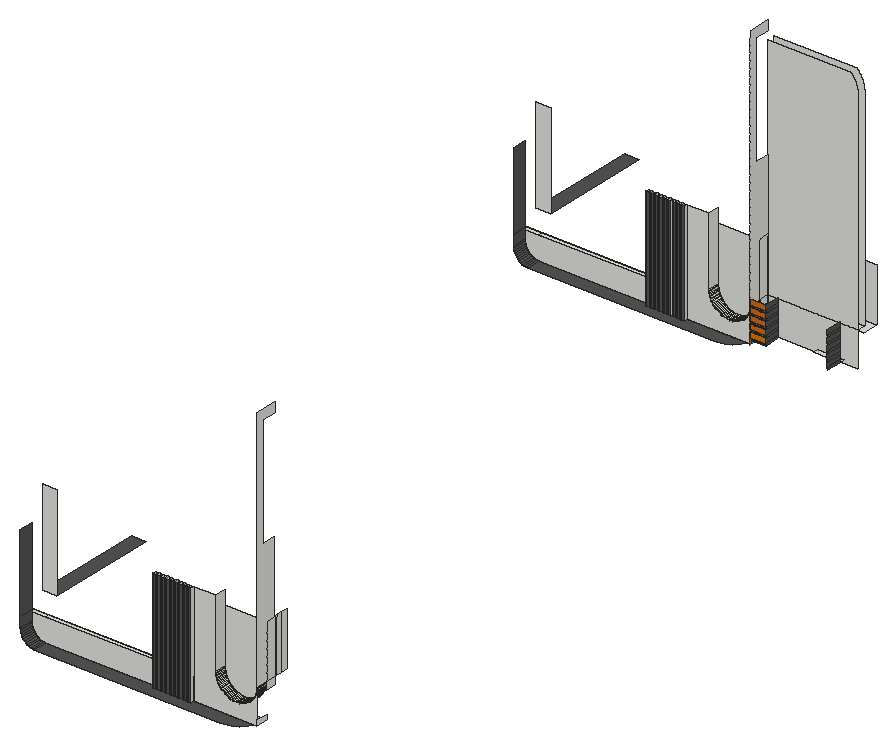
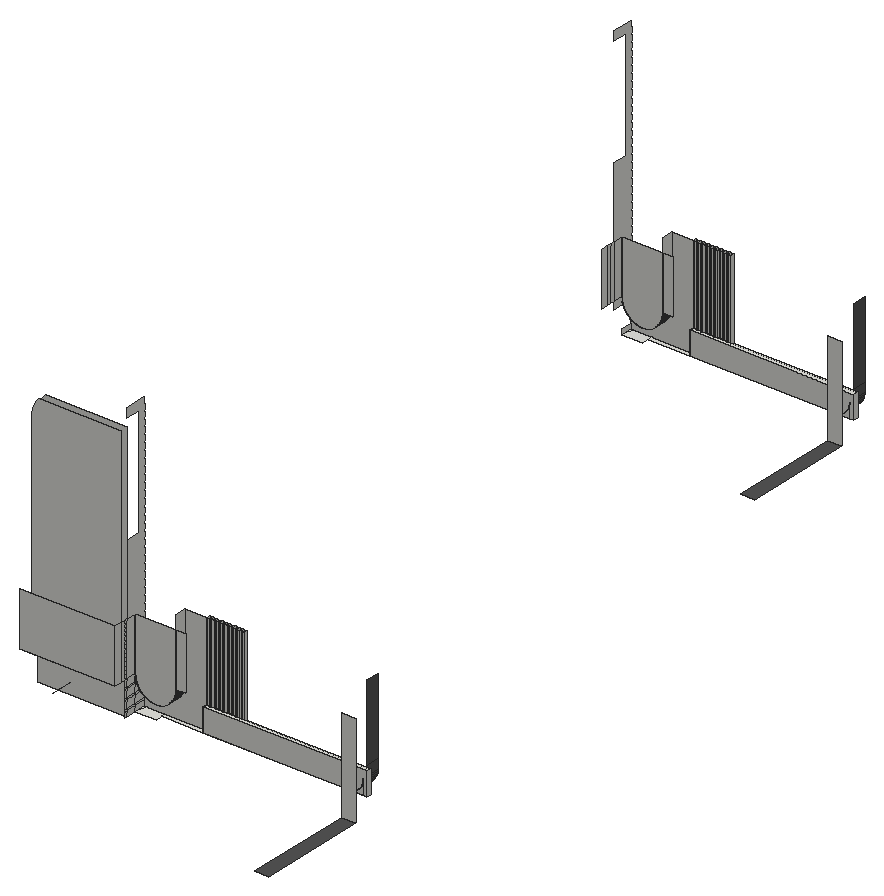
# SketchUp Ruby script. Lengths in inches.
U = 1.inch
M = Sketchup.active_model
def pt(a) = Geom::Point3d.new(a.map { |v| v * U })
def face(e, loops, mat)
  f = e.add_face(loops[0].map { |a| pt(a) })
  loops[1..].each { |l| e.add_face(l.map { |a| pt(a) }).erase! }
  f.material = f.back_material = mat if mat
  f
end
# faces: each face lists its corners as indices into pts; further lists are holes
def faces(e, pts, list, mat = nil) = list.each { |f| face(e, (f[0].is_a?(Array) ? f : [f]).map { |l| l.map { |i| pts[i] } }, mat) }
# xy, xz, yz: faces in a plane at the given z, y or x. An outline is a flat list of corners, or four numbers for a rectangle; further outlines are holes
def ring(l) = l.size == 4 ? [[l[0], l[1]], [l[2], l[1]], [l[2], l[3]], [l[0], l[3]]] : l.each_slice(2).to_a
def flat(e, list, mat, &to3) = list.each { |f| face(e, (f[0].is_a?(Array) ? f : [f]).map { |l| ring(l).map { |u, v| to3.(u, v) } }, mat) }
def xy(e, z, list, mat = nil) = flat(e, list, mat) { |x, y| [x, y, z] }
def xz(e, y, list, mat = nil) = flat(e, list, mat) { |x, z| [x, y, z] }
def yz(e, x, list, mat = nil) = flat(e, list, mat) { |y, z| [x, y, z] }
def lines(e, pts, list) = list.each { |a, b| e.add_line(pt(pts[a]), pt(pts[b])) }
# prism: a flat outline (further loops are holes) pulled along v
def prism(e, loops, v, mat = nil)
  f = face(e, loops, mat); d = Geom::Vector3d.new(v.map { |x| x * U })
  f.pushpull(f.normal.samedirection?(d) ? d.length : -d.length)
end
def box(e, o, s, mat = nil) = prism(e, [[o, [o[0] + s[0], o[1], o[2]], [o[0] + s[0], o[1] + s[1], o[2]], [o[0], o[1] + s[1], o[2]]]], [0, 0, s[2]], mat)
def at(x, y, z, deg = 0) = Geom::Transformation.translation(pt([x, y, z])) * Geom::Transformation.rotation(ORIGIN, Z_AXIS, deg.degrees)
def axes(o, x, y, z) = Geom::Transformation.new([*x, 0, *y, 0, *z, 0, *pt(o).to_a, 1])
def part(name) = M.definitions.add(name)
# library, detail: a bought-in or finely detailed component or shape, given as its bounding box
def library(name, o, s) = part(name).tap { |d| box(d.entities, o, s) }
def detail(e, o, s) = box(e.add_group.entities, o, s)
def put(e, d, t, mat = nil) = e.add_instance(d, t).tap { |i| i.material = mat if mat }
def group(e, t, mat = nil) = e.add_group.tap { |g| g.transformation = t; g.material = mat if mat }.entities
root = M.entities
M.materials.add("[0039_DarkOrange]").color = [219, 120, 0]
M.materials.add("[0041_Chocolate]").color = [210, 105, 30]
M.materials.add("[Color M06]").color = [84, 84, 84]
xy(root,141.26,[[675.54,281.47,692.98,285.84],[692.98,281.47,836,285.84],[836,281.47,876.59,285.84],[876.59,281.47,894.57,281.47,895.33,283,896.37,286.06,897,289.23,897.21,292.45,876.59,292.45],[894.57,281.47,895.33,283,896.37,286.06,897,289.23,897.21,292.45,897.21,281.47],
  [598.85,972.36,616.29,976.74],[616.29,972.36,759.32,976.74],[759.32,972.36,799.9,976.74],[799.9,972.36,817.89,972.36,818.64,973.89,819.68,976.95,820.3125,980.12,820.52,983.34,799.9,983.34],[817.89,972.36,818.64,973.89,819.68,976.95,820.3125,980.12,820.52,983.34,820.52,972.36]])
xy(root,141.26,[[692.98,267.75,872.51,267.75,875.73,267.96,878.9,268.59,881.96,269.63,884.86,271.06,887.55,272.85,889.98,274.98,892.11,277.41,893.9,280.1,894.57,281.47,836,281.47,836,278.34,832.88,278.34,832.88,281.47,831.63,281.47,831.63,278.34,828.5,278.34,828.5,281.47,827.44,281.47,827.44,278.34,824.32,278.34,824.32,281.47,823.25,281.47,823.25,278.34,820.13,278.34,820.13,281.47,819.07,281.47,819.07,278.34,815.94,278.34,815.94,281.47,814.88,281.47,814.88,278.34,811.75,278.34,811.75,281.47,810.63,281.47,810.63,278.34,807.5,278.34,807.5,281.47,806.38,281.47,806.38,278.34,803.25,278.34,803.25,281.47,802.13,281.47,802.13,278.34,799,278.34,799,281.47,692.98,281.47],[616.29,958.64,795.82,958.64,799.05,958.86,802.22,959.49,805.28,960.52,808.17,961.95,810.86,963.75,813.29,965.88,815.42,968.31,817.21,970.99,817.89,972.36,759.32,972.36,759.32,969.24,756.19,969.24,756.19,972.36,754.94,972.36,754.94,969.24,751.82,969.24,751.82,972.36,750.75,972.36,750.75,969.24,747.63,969.24,747.63,972.36,746.57,972.36,746.57,969.24,743.44,969.24,743.44,972.36,742.38,972.36,742.38,969.24,739.25,969.24,739.25,972.36,738.19,972.36,738.19,969.24,735.07,969.24,735.07,972.36,733.94,972.36,733.94,969.24,730.82,969.24,730.82,972.36,729.69,972.36,729.69,969.24,726.57,969.24,726.57,972.36,725.44,972.36,725.44,969.24,722.32,969.24,722.32,972.36,616.29,972.36]],"[Color M06]")
xy(root,145.27,[[870.3,986.55,895.48,991.24]])
xy(root,145.27,[[820.52,971.36,835.91,972.36]],"[0039_DarkOrange]")
xy(root,147.375,[[820.52,971.36,835.91,972.36]],"[0039_DarkOrange]")
xy(root,148.66,[[648.9,333.33,662.61,439.98],[572.21,1024.22,585.93,1130.875]],"[Color M06]")
xy(root,152.33,[[820.52,971.36,835.91,972.36]],"[0039_DarkOrange]")
xy(root,154.4375,[[820.52,971.36,835.91,972.36]],"[0041_Chocolate]")
xy(root,159.39,[[820.52,971.36,835.91,972.36]],"[0041_Chocolate]")
xy(root,161.5,[[820.52,971.36,835.91,972.36]],"[0041_Chocolate]")
xy(root,163.7,[[675.54,281.47,692.98,285.84],[692.98,281.47,836,285.84],[598.85,972.36,616.29,976.74],[616.29,972.36,759.32,976.74]])
xy(root,166.45,[[820.52,971.36,835.91,972.36]],"[0041_Chocolate]")
xy(root,168.5625,[[820.52,971.36,835.91,972.36]],"[0041_Chocolate]")
xy(root,173.52,[[820.52,971.36,835.91,972.36]],"[0041_Chocolate]")
xy(root,174.51,[[820.52,993.35,907.49,1001.16],[907.49,993.35,907.49,1001.16,820.52,1001.16,820.52,1008.21,913.34,1008.21,913.34,993.35]])
xy(root,175.625,[[820.52,971.36,835.91,972.36]],"[0041_Chocolate]")
xz(root,278.34,[[799,141.26,802.13,240.16],[803.25,141.26,806.38,240.16],[807.5,141.26,810.63,240.16],[811.75,141.26,814.88,240.16],[815.94,141.26,819.07,240.16],
  [820.13,141.26,823.25,240.16],[824.32,141.26,827.44,240.16],[828.5,141.26,831.63,240.16],[832.88,141.26,836,240.16]],"[Color M06]")
xz(root,281.47,[[675.54,141.26,679.54,163.7],[679.54,141.26,692.98,141.26,691.2,141.46,689.46,141.89,687.79,142.53,686.21,143.38,684.75,144.42,683.43,145.64,682.28,147.01,681.32,148.52,680.55,150.14,679.99,151.84,679.65,153.6,679.54,155.39],[692.98,141.26,799,141.26,799,163.7,679.54,163.7,679.54,155.39,679.65,153.6,679.99,151.84,680.55,150.14,681.32,148.52,682.28,147.01,683.43,145.64,684.75,144.42,686.21,143.38,687.79,142.53,689.46,141.89,691.2,141.46],[799,141.26,802.13,163.7],[802.13,141.26,803.25,163.7],
  [803.25,141.26,806.38,163.7],[806.38,141.26,807.5,163.7],[807.5,141.26,810.63,163.7],[810.63,141.26,811.75,163.7],[811.75,141.26,814.88,163.7],
  [814.88,141.26,815.94,163.7],[815.94,141.26,819.07,163.7],[819.07,141.26,820.13,163.7],[820.13,141.26,823.25,163.7],[823.25,141.26,824.32,163.7],
  [824.32,141.26,827.44,163.7],[827.44,141.26,828.5,163.7],[828.5,141.26,831.63,163.7],[831.63,141.26,832.88,163.7],[832.88,141.26,836,163.7],
  [836,141.26,897.21,141.26,897.21,174.51,897.18,173.46,897.1,172.42,896.96,171.38,896.77,170.36,896.53,169.34,896.23,168.33,895.88,167.35,895.48,166.38,895.03,165.4375,894.53,164.52,893.99,163.625,893.39,162.76,892.76,161.93,892.08,161.14,891.36,160.38,890.6,159.66,889.8,158.98,888.97,158.34,888.11,157.75,887.22,157.2,886.3,156.7,885.36,156.25,884.39,155.85,883.4,155.5,882.4,155.21,881.38,154.96,880.35,154.77,879.32,154.64,878.27,154.55,877.23,154.53,876.18,154.55,875.14,154.64,874.1,154.77,873.07,154.96,872.05,155.21,871.05,155.5,870.07,155.85,869.1,156.25,868.15,156.7,867.23,157.2,866.34,157.75,865.48,158.34,864.65,158.98,863.85,159.66,863.1,160.38,862.375,161.14,861.7,161.93,861.06,162.76,860.47,163.625,859.92,164.52,859.42,165.4375,858.97,166.38,858.57,167.35,858.22,168.33,857.92,169.34,857.68,170.36,857.49,171.38,857.35,172.42,857.27,173.46,857.24,174.51,857.24,240.16,836,240.16],[799,163.7,802.13,240.16],[803.25,163.7,806.38,240.16],[807.5,163.7,810.63,240.16],[811.75,163.7,814.88,240.16],
  [815.94,163.7,819.07,240.16],[820.13,163.7,823.25,240.16],[824.32,163.7,827.44,240.16],[828.5,163.7,831.63,240.16],[832.88,163.7,836,240.16]])
xz(root,285.84,[[675.54,141.26,675.54,163.7,692.98,163.7,692.98,141.26,691.2,141.46,689.46,141.89,687.79,142.53,686.21,143.38,684.75,144.42,683.43,145.64,682.28,147.01,681.32,148.52,680.55,150.14,679.99,151.84,679.65,153.6,679.54,155.39,679.54,141.26],[679.54,141.26,679.54,155.39,679.65,153.6,679.99,151.84,680.55,150.14,681.32,148.52,682.28,147.01,683.43,145.64,684.75,144.42,686.21,143.38,687.79,142.53,689.46,141.89,691.2,141.46,692.98,141.26],[692.98,141.26,836,163.7]])
xz(root,292.45,[[877.23,154.53,878.27,154.55,879.32,154.64,880.35,154.77,881.38,154.96,882.4,155.21,883.4,155.5,884.39,155.85,885.36,156.25,886.3,156.7,887.22,157.2,888.11,157.75,888.97,158.34,889.8,158.98,890.6,159.66,891.36,160.38,892.08,161.14,892.76,161.93,893.39,162.76,893.99,163.625,894.53,164.52,895.03,165.4375,895.48,166.38,895.88,167.35,896.23,168.33,896.53,169.34,896.77,170.36,896.96,171.38,897.1,172.42,897.18,173.46,897.21,174.51,897.21,226.8,857.24,226.8,857.24,174.51,857.27,173.46,857.35,172.42,857.49,171.38,857.68,170.36,857.92,169.34,858.22,168.33,858.57,167.35,858.97,166.38,859.42,165.4375,859.92,164.52,860.47,163.625,861.06,162.76,861.7,161.93,862.375,161.14,863.1,160.38,863.85,159.66,864.65,158.98,865.48,158.34,866.34,157.75,867.23,157.2,868.15,156.7,869.1,156.25,870.07,155.85,871.05,155.5,872.05,155.21,873.07,154.96,874.1,154.77,875.14,154.64,876.18,154.55],[847.59,174.51,857.24,226.8]])
xz(root,333.33,[[648.9,148.66,662.61,240.16]])
xz(root,969.24,[[722.32,141.26,725.44,240.16],[726.57,141.26,729.69,240.16],[730.82,141.26,733.94,240.16],[735.07,141.26,738.19,240.16],[739.25,141.26,742.38,240.16],
  [743.44,141.26,746.57,240.16],[747.63,141.26,750.75,240.16],[751.82,141.26,754.94,240.16],[756.19,141.26,759.32,240.16]],"[Color M06]")
xz(root,971.36,[[820.52,147.375,835.91,152.33]],"[0039_DarkOrange]")
xz(root,971.36,[[820.52,154.4375,835.91,159.39],[820.52,161.5,835.91,166.45],[820.52,168.5625,835.91,173.52],[820.52,175.625,835.91,180.58]],"[0041_Chocolate]")
xz(root,972.36,[[598.85,141.26,602.85,163.7],[602.85,141.26,616.29,141.26,614.51,141.46,612.77,141.89,611.1,142.53,609.52,143.38,608.0625,144.42,606.75,145.64,605.6,147.01,604.63,148.52,603.86,150.14,603.3,151.84,602.96,153.6,602.85,155.39],[616.29,141.26,722.32,141.26,722.32,163.7,602.85,163.7,602.85,155.39,602.96,153.6,603.3,151.84,603.86,150.14,604.63,148.52,605.6,147.01,606.75,145.64,608.0625,144.42,609.52,143.38,611.1,142.53,612.77,141.89,614.51,141.46],[722.32,141.26,725.44,163.7],[725.44,141.26,726.57,163.7],
  [726.57,141.26,729.69,163.7],[729.69,141.26,730.82,163.7],[730.82,141.26,733.94,163.7],[733.94,141.26,735.07,163.7],[735.07,141.26,738.19,163.7],
  [738.19,141.26,739.25,163.7],[739.25,141.26,742.38,163.7],[742.38,141.26,743.44,163.7],[743.44,141.26,746.57,163.7],[746.57,141.26,747.63,163.7],
  [747.63,141.26,750.75,163.7],[750.75,141.26,751.82,163.7],[751.82,141.26,754.94,163.7],[754.94,141.26,756.19,163.7],[756.19,141.26,759.32,163.7],
  [759.32,141.26,820.52,141.26,820.52,174.51,820.5,173.46,820.41,172.42,820.28,171.38,820.09,170.36,819.84,169.34,819.55,168.33,819.2,167.35,818.8,166.38,818.35,165.4375,817.85,164.52,817.3,163.625,816.71,162.76,816.07,161.93,815.39,161.14,814.67,160.38,813.91,159.66,813.12,158.98,812.29,158.34,811.42,157.75,810.53,157.2,809.61,156.7,808.67,156.25,807.7,155.85,806.71,155.5,805.71,155.21,804.69,154.96,803.67,154.77,802.63,154.64,801.59,154.55,800.54,154.53,799.49,154.55,798.45,154.64,797.41,154.77,796.38,154.96,795.37,155.21,794.36,155.5,793.38,155.85,792.41,156.25,791.47,156.7,790.55,157.2,789.66,157.75,788.79,158.34,787.96,158.98,787.17,159.66,786.41,160.38,785.6875,161.14,785.01,161.93,784.37,162.76,783.78,163.625,783.23,164.52,782.73,165.4375,782.28,166.38,781.88,167.35,781.53,168.33,781.24,169.34,780.99,170.36,780.8,171.38,780.66,172.42,780.58,173.46,780.56,174.51,780.56,240.16,759.32,240.16],[722.32,163.7,725.44,240.16],[726.57,163.7,729.69,240.16],[730.82,163.7,733.94,240.16],[735.07,163.7,738.19,240.16],
  [739.25,163.7,742.38,240.16],[743.44,163.7,746.57,240.16],[747.63,163.7,750.75,240.16],[751.82,163.7,754.94,240.16],[756.19,163.7,759.32,240.16]])
xz(root,972.36,[[820.52,145.27,835.91,147.375]],"[0039_DarkOrange]")
xz(root,972.36,[[820.52,152.33,835.91,154.4375],[820.52,159.39,835.91,161.5],[820.52,166.45,835.91,168.5625],[820.52,173.52,835.91,175.625]],"[0041_Chocolate]")
xz(root,976.74,[[598.85,141.26,598.85,163.7,616.29,163.7,616.29,141.26,614.51,141.46,612.77,141.89,611.1,142.53,609.52,143.38,608.0625,144.42,606.75,145.64,605.6,147.01,604.63,148.52,603.86,150.14,603.3,151.84,602.96,153.6,602.85,155.39,602.85,141.26],[602.85,141.26,602.85,155.39,602.96,153.6,603.3,151.84,603.86,150.14,604.63,148.52,605.6,147.01,606.75,145.64,608.0625,144.42,609.52,143.38,611.1,142.53,612.77,141.89,614.51,141.46,616.29,141.26],[616.29,141.26,759.32,163.7]])
xz(root,983.34,[[800.54,154.53,801.59,154.55,802.63,154.64,803.67,154.77,804.69,154.96,805.71,155.21,806.71,155.5,807.7,155.85,808.67,156.25,809.61,156.7,810.53,157.2,811.42,157.75,812.29,158.34,813.12,158.98,813.91,159.66,814.67,160.38,815.39,161.14,816.07,161.93,816.71,162.76,817.3,163.625,817.85,164.52,818.35,165.4375,818.8,166.38,819.2,167.35,819.55,168.33,819.84,169.34,820.09,170.36,820.28,171.38,820.41,172.42,820.5,173.46,820.52,174.51,820.52,226.8,780.56,226.8,780.56,174.51,780.58,173.46,780.66,172.42,780.8,171.38,780.99,170.36,781.24,169.34,781.53,168.33,781.88,167.35,782.28,166.38,782.73,165.4375,783.23,164.52,783.78,163.625,784.37,162.76,785.01,161.93,785.6875,161.14,786.41,160.38,787.17,159.66,787.96,158.98,788.79,158.34,789.66,157.75,790.55,157.2,791.47,156.7,792.41,156.25,793.38,155.85,794.36,155.5,795.37,155.21,796.38,154.96,797.41,154.77,798.45,154.64,799.49,154.55],[770.9,174.51,780.56,226.8]])
xz(root,993.35,[[820.52,141.26,907.49,174.51],[820.52,174.51,907.49,174.51,907.49,376.875,907.48,377.55,907.46,378.22,907.41,378.9,907.35,379.57,907.27,380.24,907.17,380.9,907.06,381.57,906.93,382.23,906.78,382.89,906.61,383.54,906.59,383.64,906.43,384.19,906.23,384.84,906.01,385.47,905.91,385.76,905.78,386.11,905.53,386.73,905.26,387.35,904.98,387.96,904.68,388.57,904.37,389.17,904.04,389.76,903.7,390.33,903.34,390.9,902.96,391.47,902.57,392.02,902.17,392.56,901.75,393.09,901.71,393.14,901.32,393.6,900.875,394.11,900.42,394.61,899.95,395.09,899.77,395.26,820.52,395.26]])
xz(root,1001.16,[[820.52,174.51,820.52,395.26,899.77,395.26,899.95,395.09,900.42,394.61,900.875,394.11,901.32,393.6,901.71,393.14,901.75,393.09,902.17,392.56,902.57,392.02,902.96,391.47,903.34,390.9,903.7,390.33,904.04,389.76,904.37,389.17,904.68,388.57,904.98,387.96,905.26,387.35,905.53,386.73,905.78,386.11,905.91,385.76,906.01,385.47,906.23,384.84,906.43,384.19,906.59,383.64,906.61,383.54,906.78,382.89,906.93,382.23,907.06,381.57,907.17,380.9,907.27,380.24,907.35,379.57,907.41,378.9,907.46,378.22,907.48,377.55,907.49,376.875,907.49,174.51]])
xz(root,1008.21,[[820.52,174.51,913.34,226.8]])
xz(root,1024.22,[[572.21,148.66,585.93,240.16]])
yz(root,598.85,[[972.36,141.26,976.74,163.7]])
yz(root,602.85,[[958.64,155.39,972.36,164.97],[958.64,164.97,972.36,240.16]],"[Color M06]")
yz(root,675.54,[[281.47,141.26,285.84,163.7]])
yz(root,679.54,[[267.75,155.39,281.47,164.97],[267.75,164.97,281.47,240.16]],"[Color M06]")
yz(root,722.32,[[969.24,141.26,972.36,240.16]])
yz(root,725.44,[[969.24,141.26,972.36,240.16]])
yz(root,726.57,[[969.24,141.26,972.36,240.16]])
yz(root,729.69,[[969.24,141.26,972.36,240.16]])
yz(root,730.82,[[969.24,141.26,972.36,240.16]])
yz(root,733.94,[[969.24,141.26,972.36,240.16]])
yz(root,735.07,[[969.24,141.26,972.36,240.16]])
yz(root,738.19,[[969.24,141.26,972.36,240.16]])
yz(root,739.25,[[969.24,141.26,972.36,240.16]])
yz(root,742.38,[[969.24,141.26,972.36,240.16]])
yz(root,743.44,[[969.24,141.26,972.36,240.16]])
yz(root,746.57,[[969.24,141.26,972.36,240.16]])
yz(root,747.63,[[969.24,141.26,972.36,240.16]])
yz(root,750.75,[[969.24,141.26,972.36,240.16]])
yz(root,751.82,[[969.24,141.26,972.36,240.16]])
yz(root,754.94,[[969.24,141.26,972.36,240.16]])
yz(root,756.19,[[969.24,141.26,972.36,240.16]])
yz(root,759.32,[[969.24,141.26,972.36,240.16],[972.36,141.26,976.74,163.7]])
yz(root,780.56,[[972.36,174.51,983.34,240.16]])
yz(root,799,[[278.34,141.26,281.47,240.16]])
yz(root,802.13,[[278.34,141.26,281.47,240.16]])
yz(root,803.25,[[278.34,141.26,281.47,240.16]])
yz(root,806.38,[[278.34,141.26,281.47,240.16]])
yz(root,807.5,[[278.34,141.26,281.47,240.16]])
yz(root,810.63,[[278.34,141.26,281.47,240.16]])
yz(root,811.75,[[278.34,141.26,281.47,240.16]])
yz(root,814.88,[[278.34,141.26,281.47,240.16]])
yz(root,815.94,[[278.34,141.26,281.47,240.16]])
yz(root,819.07,[[278.34,141.26,281.47,240.16]])
yz(root,820.13,[[278.34,141.26,281.47,240.16]])
yz(root,820.52,[[972.36,141.26,983.34,146.14],[983.34,141.26,993.35,146.14],[993.35,141.26,996.48,146.14],[972.36,146.14,983.34,148.26],[983.34,146.14,993.35,148.26],
  [993.35,146.14,996.48,148.26],[972.36,148.26,983.34,155.64],[983.34,148.26,993.35,155.64],[993.35,148.26,996.48,155.64],[972.36,155.64,983.34,157.76],
  [983.34,155.64,993.35,157.76],[993.35,155.64,996.48,157.76],[972.36,157.76,983.34,165.14],[983.34,157.76,993.35,165.14],[993.35,157.76,996.48,165.14],
  [972.36,165.14,983.34,167.26],[983.34,165.14,993.35,167.26],[993.35,165.14,996.48,167.26],[972.36,167.26,983.34,174.51],[983.34,167.26,993.35,174.51],
  [993.35,167.26,996.48,174.51],[972.36,174.51,972.36,175.625,971.36,175.625,971.36,180.58,972.36,180.58,972.36,182.6875,971.36,182.6875,971.36,187.64,972.36,187.64,972.36,189.75,971.36,189.75,971.36,194.7,972.36,194.7,972.36,196.8125,971.36,196.8125,971.36,201.77,972.36,201.77,972.36,203.875,971.36,203.875,971.36,208.83,972.36,208.83,972.36,210.9375,971.36,210.9375,971.36,215.89,972.36,215.89,972.36,218,971.36,218,971.36,222.95,972.36,222.95,972.36,225.0625,971.36,225.0625,971.36,230.02,972.36,230.02,972.36,232.125,971.36,232.125,971.36,237.08,972.36,237.08,972.36,239.1875,971.36,239.1875,971.36,244.14,972.36,244.14,972.36,246.25,971.36,246.25,971.36,251.2,972.36,251.2,972.36,253.3125,971.36,253.3125,971.36,258.27,972.36,258.27,972.36,260.375,971.36,260.375,971.36,265.33,972.36,265.33,972.36,267.4375,971.36,267.4375,971.36,272.39,972.36,272.39,972.36,274.5,971.36,274.5,971.36,279.45,972.36,279.45,972.36,281.5625,971.36,281.5625,971.36,286.52,972.36,286.52,972.36,288.625,971.36,288.625,971.36,293.58,972.36,293.58,972.36,295.6875,971.36,295.6875,971.36,300.64,972.36,300.64,972.36,302.75,971.36,302.75,971.36,307.7,972.36,307.7,972.36,309.8125,971.36,309.8125,971.36,314.77,972.36,314.77,972.36,316.875,971.36,316.875,971.36,321.83,972.36,321.83,972.36,323.9375,971.36,323.9375,971.36,328.89,972.36,328.89,972.36,331,971.36,331,971.36,335.95,972.36,335.95,972.36,338.0625,971.36,338.0625,971.36,343.02,972.36,343.02,972.36,345.125,971.36,345.125,971.36,350.08,972.36,350.08,972.36,352.1875,971.36,352.1875,971.36,357.14,972.36,357.14,972.36,359.25,971.36,359.25,971.36,364.2,972.36,364.2,972.36,366.3125,971.36,366.3125,971.36,371.27,972.36,371.27,972.36,373.1875,971.36,373.1875,971.36,378.14,972.36,378.14,972.36,380.0625,971.36,380.0625,971.36,385.02,972.36,385.02,972.36,386.9375,971.36,386.9375,971.36,391.89,972.36,391.89,972.36,393.8125,971.36,393.8125,971.36,398.77,972.36,398.77,972.36,400.6875,971.36,400.6875,971.36,405.64,972.36,405.64,972.36,411.82,993.35,411.82,993.35,402.64,978.84,402.64,978.84,295.72,992.96,295.72,992.96,226.8,983.34,226.8,983.34,174.51],[983.34,174.51,993.35,226.8],[993.35,174.51,996.48,226.8],[996.48,174.51,1001.16,226.8],
  [1001.16,174.51,1008.21,226.8]])
yz(root,820.52,[[971.36,141.26,972.36,145.27],[971.36,147.375,972.36,148.26],[971.36,148.26,972.36,152.33]],"[0039_DarkOrange]")
yz(root,820.52,[[971.36,154.4375,972.36,155.64],[971.36,155.64,972.36,157.76],[971.36,157.76,972.36,159.39],[971.36,161.5,972.36,165.14],[971.36,165.14,972.36,166.45],
  [971.36,168.5625,972.36,173.52]],"[0041_Chocolate]")
yz(root,823.25,[[278.34,141.26,281.47,240.16]])
yz(root,824.32,[[278.34,141.26,281.47,240.16]])
yz(root,827.44,[[278.34,141.26,281.47,240.16]])
yz(root,828.5,[[278.34,141.26,281.47,240.16]])
yz(root,831.63,[[278.34,141.26,281.47,240.16]])
yz(root,832.88,[[278.34,141.26,281.47,240.16]])
yz(root,835.91,[[972.36,145.27,986.55,147.375],[971.36,147.375,986.55,152.33],[972.36,152.33,986.55,154.4375],[971.36,154.4375,986.55,159.39],[972.36,159.39,986.55,161.5],
  [971.36,161.5,986.55,166.45],[972.36,166.45,986.55,168.5625],[971.36,168.5625,986.55,173.52],[972.36,173.52,986.55,175.625],[971.36,175.625,986.55,180.58]],"[Color M06]")
yz(root,836,[[278.34,141.26,281.47,240.16],[281.47,141.26,285.84,163.7]])
yz(root,857.24,[[281.47,174.51,292.45,240.16]])
yz(root,895.48,[[972.36,145.27,986.55,147.375],[971.36,147.375,986.55,152.33],[972.36,152.33,986.55,154.4375],[971.36,154.4375,986.55,159.39],[972.36,159.39,986.55,161.5],
  [971.36,161.5,986.55,166.45],[972.36,166.45,986.55,168.5625],[971.36,168.5625,986.55,173.52],[972.36,173.52,986.55,175.625],[971.36,175.625,986.55,180.58]],"[Color M06]")
yz(root,897.21,[[281.47,141.26,292.45,146.14],[292.45,167.26,302.46,174.51],[281.47,174.51,281.47,175.625,280.47,175.625,280.47,180.58,281.47,180.58,281.47,182.6875,280.47,182.6875,280.47,187.64,281.47,187.64,281.47,189.75,280.47,189.75,280.47,194.7,281.47,194.7,281.47,196.8125,280.47,196.8125,280.47,201.77,281.47,201.77,281.47,203.875,280.47,203.875,280.47,208.83,281.47,208.83,281.47,210.9375,280.47,210.9375,280.47,215.89,281.47,215.89,281.47,218,280.47,218,280.47,222.95,281.47,222.95,281.47,225.0625,280.47,225.0625,280.47,230.02,281.47,230.02,281.47,232.125,280.47,232.125,280.47,237.08,281.47,237.08,281.47,239.1875,280.47,239.1875,280.47,244.14,281.47,244.14,281.47,246.25,280.47,246.25,280.47,251.2,281.47,251.2,281.47,253.3125,280.47,253.3125,280.47,258.27,281.47,258.27,281.47,260.375,280.47,260.375,280.47,265.33,281.47,265.33,281.47,267.4375,280.47,267.4375,280.47,272.39,281.47,272.39,281.47,274.5,280.47,274.5,280.47,279.45,281.47,279.45,281.47,281.5625,280.47,281.5625,280.47,286.52,281.47,286.52,281.47,288.625,280.47,288.625,280.47,293.58,281.47,293.58,281.47,295.6875,280.47,295.6875,280.47,300.64,281.47,300.64,281.47,302.75,280.47,302.75,280.47,307.7,281.47,307.7,281.47,309.8125,280.47,309.8125,280.47,314.77,281.47,314.77,281.47,316.875,280.47,316.875,280.47,321.83,281.47,321.83,281.47,323.9375,280.47,323.9375,280.47,328.89,281.47,328.89,281.47,331,280.47,331,280.47,335.95,281.47,335.95,281.47,338.0625,280.47,338.0625,280.47,343.02,281.47,343.02,281.47,345.125,280.47,345.125,280.47,350.08,281.47,350.08,281.47,352.1875,280.47,352.1875,280.47,357.14,281.47,357.14,281.47,359.25,280.47,359.25,280.47,364.2,281.47,364.2,281.47,366.3125,280.47,366.3125,280.47,371.27,281.47,371.27,281.47,373.1875,280.47,373.1875,280.47,378.14,281.47,378.14,281.47,380.0625,280.47,380.0625,280.47,385.02,281.47,385.02,281.47,386.9375,280.47,386.9375,280.47,391.89,281.47,391.89,281.47,393.8125,280.47,393.8125,280.47,398.77,281.47,398.77,281.47,400.6875,280.47,400.6875,280.47,405.64,281.47,405.64,281.47,411.82,302.46,411.82,302.46,402.64,287.95,402.64,287.95,295.72,302.0625,295.72,302.0625,226.8,292.45,226.8,292.45,174.51],[292.45,174.51,302.46,226.8],[302.46,174.51,305.58,226.8],
  [305.58,174.51,310.27,226.8],[310.27,174.51,317.3125,226.8]])
p = [[691.2,267.75,141.46],[692.98,267.75,141.26],[692.98,281.47,141.26],[691.2,281.47,141.46],[692.98,285.84,141.26],[691.2,285.84,141.46],
  [614.51,958.64,141.46],[616.29,958.64,141.26],[616.29,972.36,141.26],[614.51,972.36,141.46],[616.29,976.74,141.26],[614.51,976.74,141.46],
  [689.46,267.75,141.89],[689.46,281.47,141.89],[689.46,285.84,141.89],[612.77,958.64,141.89],[612.77,972.36,141.89],[612.77,976.74,141.89],
  [687.79,267.75,142.53],[687.79,281.47,142.53],[687.79,285.84,142.53],[611.1,958.64,142.53],[611.1,972.36,142.53],[611.1,976.74,142.53],
  [686.21,267.75,143.38],[686.21,281.47,143.38],[686.21,285.84,143.38],[609.52,958.64,143.38],[609.52,972.36,143.38],[609.52,976.74,143.38],
  [684.75,267.75,144.42],[684.75,281.47,144.42],[684.75,285.84,144.42],[608.0625,958.64,144.42],[608.0625,972.36,144.42],[608.0625,976.74,144.42],
  [683.43,267.75,145.64],[683.43,281.47,145.64],[683.43,285.84,145.64],[606.75,958.64,145.64],[606.75,972.36,145.64],[606.75,976.74,145.64],
  [682.28,267.75,147.01],[682.28,281.47,147.01],[682.28,285.84,147.01],[605.6,958.64,147.01],[605.6,972.36,147.01],[605.6,976.74,147.01],
  [681.32,267.75,148.52],[681.32,281.47,148.52],[681.32,285.84,148.52],[604.63,958.64,148.52],[604.63,972.36,148.52],[604.63,976.74,148.52],
  [680.55,267.75,150.14],[680.55,281.47,150.14],[680.55,285.84,150.14],[603.86,958.64,150.14],[603.86,972.36,150.14],[603.86,976.74,150.14],
  [679.99,267.75,151.84],[679.99,281.47,151.84],[679.99,285.84,151.84],[603.3,958.64,151.84],[603.3,972.36,151.84],[603.3,976.74,151.84],
  [679.65,267.75,153.6],[679.65,281.47,153.6],[679.65,285.84,153.6],[602.96,958.64,153.6],[602.96,972.36,153.6],[602.96,976.74,153.6],
  [679.54,267.75,155.39],[679.54,281.47,155.39],[679.54,285.84,155.39],[602.85,958.64,155.39],[602.85,972.36,155.39],[602.85,976.74,155.39],
  [877.23,292.45,154.53],[876.18,292.45,154.55],[876.18,281.47,154.55],[877.23,281.47,154.53],[878.27,292.45,154.55],[878.27,281.47,154.55],
  [800.54,983.34,154.53],[799.49,983.34,154.55],[799.49,972.36,154.55],[800.54,972.36,154.53],[801.59,983.34,154.55],[801.59,972.36,154.55],
  [875.14,292.45,154.64],[874.1,292.45,154.77],[874.1,281.47,154.77],[875.14,281.47,154.64],[879.32,292.45,154.64],[879.32,281.47,154.64],
  [880.35,292.45,154.77],[880.35,281.47,154.77],[798.45,983.34,154.64],[797.41,983.34,154.77],[797.41,972.36,154.77],[798.45,972.36,154.64],
  [802.63,983.34,154.64],[802.63,972.36,154.64],[803.67,983.34,154.77],[803.67,972.36,154.77],[873.07,292.45,154.96],[873.07,281.47,154.96],
  [881.38,292.45,154.96],[881.38,281.47,154.96],[796.38,983.34,154.96],[796.38,972.36,154.96],[804.69,983.34,154.96],[804.69,972.36,154.96],
  [872.05,292.45,155.21],[872.05,281.47,155.21],[882.4,292.45,155.21],[882.4,281.47,155.21],[795.37,983.34,155.21],[795.37,972.36,155.21],
  [805.71,983.34,155.21],[805.71,972.36,155.21],[871.05,292.45,155.5],[871.05,281.47,155.5],[883.4,292.45,155.5],[883.4,281.47,155.5],
  [794.36,983.34,155.5],[794.36,972.36,155.5],[806.71,983.34,155.5],[806.71,972.36,155.5],[870.07,292.45,155.85],[870.07,281.47,155.85],
  [884.39,292.45,155.85],[884.39,281.47,155.85],[793.38,983.34,155.85],[793.38,972.36,155.85],[807.7,983.34,155.85],[807.7,972.36,155.85],
  [869.1,292.45,156.25],[869.1,281.47,156.25],[885.36,292.45,156.25],[885.36,281.47,156.25],[792.41,983.34,156.25],[792.41,972.36,156.25],
  [808.67,983.34,156.25],[808.67,972.36,156.25],[868.15,292.45,156.7],[868.15,281.47,156.7],[886.3,292.45,156.7],[886.3,281.47,156.7],
  [791.47,983.34,156.7],[791.47,972.36,156.7],[809.61,983.34,156.7],[809.61,972.36,156.7],[867.23,292.45,157.2],[867.23,281.47,157.2],
  [887.22,292.45,157.2],[887.22,281.47,157.2],[790.55,983.34,157.2],[790.55,972.36,157.2],[810.53,983.34,157.2],[810.53,972.36,157.2],
  [866.34,292.45,157.75],[866.34,281.47,157.75],[888.11,292.45,157.75],[888.11,281.47,157.75],[789.66,983.34,157.75],[789.66,972.36,157.75],
  [811.42,983.34,157.75],[811.42,972.36,157.75],[865.48,292.45,158.34],[865.48,281.47,158.34],[888.97,292.45,158.34],[888.97,281.47,158.34],
  [788.79,983.34,158.34],[788.79,972.36,158.34],[812.29,983.34,158.34],[812.29,972.36,158.34],[864.65,292.45,158.98],[864.65,281.47,158.98],
  [889.8,292.45,158.98],[889.8,281.47,158.98],[787.96,983.34,158.98],[787.96,972.36,158.98],[813.12,983.34,158.98],[813.12,972.36,158.98],
  [863.85,292.45,159.66],[863.85,281.47,159.66],[890.6,292.45,159.66],[890.6,281.47,159.66],[787.17,983.34,159.66],[787.17,972.36,159.66],
  [813.91,983.34,159.66],[813.91,972.36,159.66],[863.1,292.45,160.38],[863.1,281.47,160.38],[891.36,292.45,160.38],[891.36,281.47,160.38],
  [786.41,983.34,160.38],[786.41,972.36,160.38],[814.67,983.34,160.38],[814.67,972.36,160.38],[862.375,292.45,161.14],[862.375,281.47,161.14],
  [892.08,292.45,161.14],[892.08,281.47,161.14],[785.6875,983.34,161.14],[785.6875,972.36,161.14],[815.39,983.34,161.14],[815.39,972.36,161.14],
  [861.7,292.45,161.93],[861.7,281.47,161.93],[892.76,292.45,161.93],[892.76,281.47,161.93],[785.01,983.34,161.93],[785.01,972.36,161.93],
  [816.07,983.34,161.93],[816.07,972.36,161.93],[861.06,292.45,162.76],[861.06,281.47,162.76],[893.39,292.45,162.76],[893.39,281.47,162.76],
  [784.37,983.34,162.76],[784.37,972.36,162.76],[816.71,983.34,162.76],[816.71,972.36,162.76],[860.47,292.45,163.625],[860.47,281.47,163.625],
  [893.99,292.45,163.625],[893.99,281.47,163.625],[783.78,983.34,163.625],[783.78,972.36,163.625],[817.3,983.34,163.625],[817.3,972.36,163.625],
  [859.92,292.45,164.52],[859.92,281.47,164.52],[894.53,292.45,164.52],[894.53,281.47,164.52],[783.23,983.34,164.52],[783.23,972.36,164.52],
  [817.85,983.34,164.52],[817.85,972.36,164.52],[859.42,292.45,165.4375],[859.42,281.47,165.4375],[895.03,292.45,165.4375],[895.03,281.47,165.4375],
  [782.73,983.34,165.4375],[782.73,972.36,165.4375],[818.35,983.34,165.4375],[818.35,972.36,165.4375],[858.97,292.45,166.38],[858.97,281.47,166.38],
  [895.48,292.45,166.38],[895.48,281.47,166.38],[782.28,983.34,166.38],[782.28,972.36,166.38],[818.8,983.34,166.38],[818.8,972.36,166.38],
  [858.57,292.45,167.35],[858.57,281.47,167.35],[895.88,292.45,167.35],[895.88,281.47,167.35],[781.88,983.34,167.35],[781.88,972.36,167.35],
  [819.2,983.34,167.35],[819.2,972.36,167.35],[858.22,292.45,168.33],[858.22,281.47,168.33],[896.23,292.45,168.33],[896.23,281.47,168.33],
  [781.53,983.34,168.33],[781.53,972.36,168.33],[819.55,983.34,168.33],[819.55,972.36,168.33],[857.92,292.45,169.34],[857.92,281.47,169.34],
  [896.53,292.45,169.34],[896.53,281.47,169.34],[781.24,983.34,169.34],[781.24,972.36,169.34],[819.84,983.34,169.34],[819.84,972.36,169.34],
  [857.68,292.45,170.36],[857.68,281.47,170.36],[896.77,292.45,170.36],[896.77,281.47,170.36],[780.99,983.34,170.36],[780.99,972.36,170.36],
  [820.09,983.34,170.36],[820.09,972.36,170.36],[857.49,292.45,171.38],[857.49,281.47,171.38],[896.96,292.45,171.38],[896.96,281.47,171.38],
  [780.8,983.34,171.38],[780.8,972.36,171.38],[820.28,983.34,171.38],[820.28,972.36,171.38],[857.35,292.45,172.42],[857.35,281.47,172.42],
  [897.1,292.45,172.42],[897.1,281.47,172.42],[780.66,983.34,172.42],[780.66,972.36,172.42],[820.41,983.34,172.42],[820.41,972.36,172.42],
  [857.27,292.45,173.46],[857.27,281.47,173.46],[897.18,292.45,173.46],[897.18,281.47,173.46],[780.58,983.34,173.46],[780.58,972.36,173.46],
  [820.5,983.34,173.46],[820.5,972.36,173.46],[857.24,292.45,174.51],[857.24,281.47,174.51],[897.21,292.45,174.51],[897.21,281.47,174.51],
  [780.56,983.34,174.51],[780.56,972.36,174.51],[820.52,983.34,174.51],[820.52,972.36,174.51],[861.07,1012.23,165.14],[861.07,1034.04,165.14]]
faces(root,p,[[0,1,2,3],[6,7,8,9],[12,0,3,13],[15,6,9,16],[18,12,13,19],[21,15,16,22],[24,18,19,25],[27,21,22,28],
  [30,24,25,31],[33,27,28,34],[36,30,31,37],[39,33,34,40],[42,36,37,43],[45,39,40,46],[48,42,43,49],[51,45,46,52],
  [54,48,49,55],[57,51,52,58],[60,54,55,61],[63,57,58,64],[66,60,61,67],[69,63,64,70],[72,66,67,73],[75,69,70,76]],"[Color M06]")
faces(root,p,[[3,2,4,5],[9,8,10,11],[13,3,5,14],[16,9,11,17],[19,13,14,20],[22,16,17,23],[25,19,20,26],[28,22,23,29],
  [31,25,26,32],[34,28,29,35],[37,31,32,38],[40,34,35,41],[43,37,38,44],[46,40,41,47],[49,43,44,50],[52,46,47,53],
  [55,49,50,56],[58,52,53,59],[61,55,56,62],[64,58,59,65],[67,61,62,68],[70,64,65,71],[73,67,68,74],[76,70,71,77],
  [78,79,80,81],[82,78,81,83],[84,85,86,87],[88,84,87,89],[90,91,92,93],[79,90,93,80],[94,82,83,95],[96,94,95,97],
  [98,99,100,101],[85,98,101,86],[102,88,89,103],[104,102,103,105],[91,106,107,92],[108,96,97,109],[99,110,111,100],[112,104,105,113],
  [106,114,115,107],[116,108,109,117],[110,118,119,111],[120,112,113,121],[114,122,123,115],[124,116,117,125],[118,126,127,119],[128,120,121,129],
  [122,130,131,123],[132,124,125,133],[126,134,135,127],[136,128,129,137],[130,138,139,131],[140,132,133,141],[134,142,143,135],[144,136,137,145],
  [138,146,147,139],[148,140,141,149],[142,150,151,143],[152,144,145,153],[146,154,155,147],[156,148,149,157],[150,158,159,151],[160,152,153,161],
  [154,162,163,155],[164,156,157,165],[158,166,167,159],[168,160,161,169],[162,170,171,163],[172,164,165,173],[166,174,175,167],[176,168,169,177],
  [170,178,179,171],[180,172,173,181],[174,182,183,175],[184,176,177,185],[178,186,187,179],[188,180,181,189],[182,190,191,183],[192,184,185,193],
  [186,194,195,187],[196,188,189,197],[190,198,199,191],[200,192,193,201],[194,202,203,195],[204,196,197,205],[198,206,207,199],[208,200,201,209],
  [202,210,211,203],[212,204,205,213],[206,214,215,207],[216,208,209,217],[210,218,219,211],[220,212,213,221],[214,222,223,215],[224,216,217,225],
  [218,226,227,219],[228,220,221,229],[222,230,231,223],[232,224,225,233],[226,234,235,227],[236,228,229,237],[230,238,239,231],[240,232,233,241],
  [234,242,243,235],[244,236,237,245],[238,246,247,239],[248,240,241,249],[242,250,251,243],[252,244,245,253],[246,254,255,247],[256,248,249,257],
  [250,258,259,251],[260,252,253,261],[254,262,263,255],[264,256,257,265],[258,266,267,259],[268,260,261,269],[262,270,271,263],[272,264,265,273],
  [266,274,275,267],[276,268,269,277],[270,278,279,271],[280,272,273,281],[274,282,283,275],[284,276,277,285],[278,286,287,279],[288,280,281,289],
  [282,290,291,283],[292,284,285,293],[286,294,295,287],[296,288,289,297],[290,298,299,291],[300,292,293,301],[294,302,303,295],[304,296,297,305],
  [298,306,307,299],[308,300,301,309],[302,310,311,303],[312,304,305,313],[306,314,315,307],[316,308,309,317],[310,318,319,311],[320,312,313,321]])
lines(root,p,[[322,323]])
